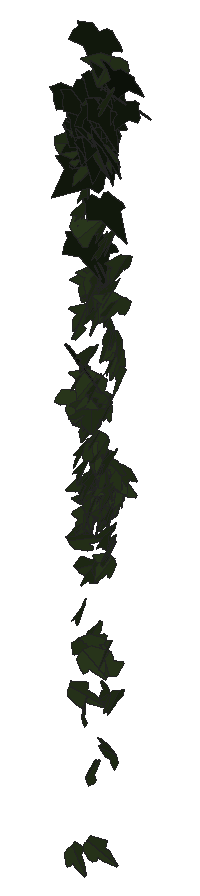
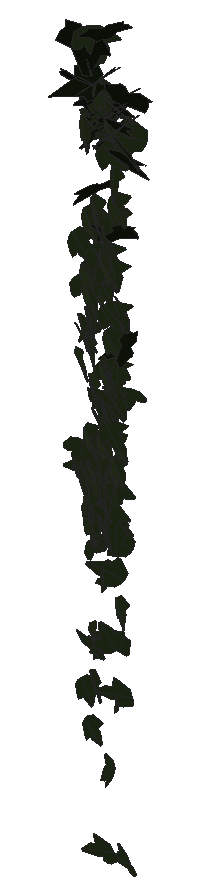
# SketchUp Ruby script. Lengths in inches.
U = 1.inch
M = Sketchup.active_model
def pt(a) = Geom::Point3d.new(a.map { |v| v * U })
def face(e, loops, mat)
  f = e.add_face(loops[0].map { |a| pt(a) })
  loops[1..].each { |l| e.add_face(l.map { |a| pt(a) }).erase! }
  f.material = f.back_material = mat if mat
  f
end
# faces: each face lists its corners as indices into pts; further lists are holes
def faces(e, pts, list, mat = nil) = list.each { |f| face(e, (f[0].is_a?(Array) ? f : [f]).map { |l| l.map { |i| pts[i] } }, mat) }
# xy, xz, yz: faces in a plane at the given z, y or x. An outline is a flat list of corners, or four numbers for a rectangle; further outlines are holes
def ring(l) = l.size == 4 ? [[l[0], l[1]], [l[2], l[1]], [l[2], l[3]], [l[0], l[3]]] : l.each_slice(2).to_a
def flat(e, list, mat, &to3) = list.each { |f| face(e, (f[0].is_a?(Array) ? f : [f]).map { |l| ring(l).map { |u, v| to3.(u, v) } }, mat) }
def xy(e, z, list, mat = nil) = flat(e, list, mat) { |x, y| [x, y, z] }
def xz(e, y, list, mat = nil) = flat(e, list, mat) { |x, z| [x, y, z] }
def yz(e, x, list, mat = nil) = flat(e, list, mat) { |y, z| [x, y, z] }
def lines(e, pts, list) = list.each { |a, b| e.add_line(pt(pts[a]), pt(pts[b])) }
# prism: a flat outline (further loops are holes) pulled along v
def prism(e, loops, v, mat = nil)
  f = face(e, loops, mat); d = Geom::Vector3d.new(v.map { |x| x * U })
  f.pushpull(f.normal.samedirection?(d) ? d.length : -d.length)
end
def box(e, o, s, mat = nil) = prism(e, [[o, [o[0] + s[0], o[1], o[2]], [o[0] + s[0], o[1] + s[1], o[2]], [o[0], o[1] + s[1], o[2]]]], [0, 0, s[2]], mat)
def at(x, y, z, deg = 0) = Geom::Transformation.translation(pt([x, y, z])) * Geom::Transformation.rotation(ORIGIN, Z_AXIS, deg.degrees)
def axes(o, x, y, z) = Geom::Transformation.new([*x, 0, *y, 0, *z, 0, *pt(o).to_a, 1])
def part(name) = M.definitions.add(name)
# library, detail: a bought-in or finely detailed component or shape, given as its bounding box
def library(name, o, s) = part(name).tap { |d| box(d.entities, o, s) }
def detail(e, o, s) = box(e.add_group.entities, o, s)
def put(e, d, t, mat = nil) = e.add_instance(d, t).tap { |i| i.material = mat if mat }
def group(e, t, mat = nil) = e.add_group.tap { |g| g.transformation = t; g.material = mat if mat }.entities
root = M.entities
M.materials.add("1026 AP 7946 SUNNY SIDE UP").color = [254, 231, 186]
M.materials.add("efeu1").color = [18, 25, 13]
M.materials.add("efeu2").color = [43, 57, 29]
c1 = part("ivyleaf_10")
p = [[0,0.5,-0.03],[-0.0625,2.02,-0.43],[-0.19,2.01,-0.46],[-0.54,1.05,-0.29],[-0.52,0.625,-0.18],[-0.83,0.76,-0.28],
  [-1.16,0.64,-0.33],[-1.15,0.33,-0.24],[-0.77,-0.39,0.02],[-0.3,-0.51,0.16],[0.04,-0.48,0.23],[-0.02,2.01,-0.4375],
  [-0.06,2.01,-0.43],[0.04,-0.49,0.23],[0.67,-0.49,0.14],[1.38,0.36,-0.2],[1.375,0.51,-0.24],[0.81,0.65,-0.19],
  [0.62,0.59,-0.15],[0.6,1.09,-0.28],[0.5,1.23,-0.31]]
faces(c1.entities,p,[[0,1,2,3,4,5,6,7,8,9,10],[11,12,0,13,14,15,16,17,18,19,20]],"efeu2")
c2 = part("ivyleaf_9")
p = [[1.54,2.16,1.25],[1.36,2.04,1.19],[-0.21,0.99,0.68],[-0.71,1.11,0.82],[-0.85,0.86,0.67],[-0.8,0.17,0.21],
  [-0.9,-0.01,0.1],[-0.67,-0.16,-0.02],[-0.08,-0.08,-0.05],[-0.03,-0.6,-0.4],[0.65,-0.88,-0.66],[0.83,-0.6,-0.49],
  [1.29,-0.42,-0.43],[1.8125,-0.07,-0.26],[1.21,0.44,0.15]]
faces(c2.entities,p,[[0,1,2,3,4,5,6,7,8,9,10,11,12,13,14]],"efeu1")
put(root,c1,axes([102.23,212.57,265.25],[0.00856,-0.04702,0.25643],[0.22762,0.20521,0.03784],[-0.32737,0.14145,0.03301]),"1026 AP 7946 SUNNY SIDE UP")
put(root,c2,axes([102.23,212.81,266.26],[-0.06893,-0.1302,-0.2167],[0.23021,0.15765,-0.1315],[0.31233,-0.14493,0.0491]),"1026 AP 7946 SUNNY SIDE UP")
put(root,c1,axes([102.46,212.81,257.53],[-0.08441,-0.19951,-0.06343],[0.03617,0.05635,-0.21239],[0.32579,-0.05795,0.00715]),"1026 AP 7946 SUNNY SIDE UP")
put(root,c1,axes([102.55,212.9,261.86],[-0.12366,-0.17588,0.12532],[-0.06753,-0.11507,-0.19904],[0.33033,-0.08937,0.00623]),"1026 AP 7946 SUNNY SIDE UP")
put(root,c1,axes([102.5,212.98,259.57],[-0.08704,-0.19196,0.06941],[-0.00761,-0.06969,-0.20573],[0.32037,-0.05381,0.01397]),"1026 AP 7946 SUNNY SIDE UP")
put(root,c1,axes([102.49,212.8,258.8],[0.03913,-0.20759,0.02258],[0.00037,-0.02323,-0.21551],[0.32842,0.02476,-0.00244]),"1026 AP 7946 SUNNY SIDE UP")
put(root,c1,axes([102.49,212.82,263.99],[0.01839,-0.23161,0.06678],[0.0176,-0.06562,-0.23917],[0.37833,0.01431,0.00788]),"1026 AP 7946 SUNNY SIDE UP")
put(root,c1,axes([102.46,212.875,258.34],[-0.19676,-0.16588,-0.03402],[0.07297,0.00464,-0.21117],[0.25545,-0.1291,0.03411]),"1026 AP 7946 SUNNY SIDE UP")
put(root,c2,axes([102.71,212.6,265.22],[-0.13705,0.20358,0.15107],[-0.11237,0.12739,-0.227],[-0.37706,-0.11196,0.01274]),"1026 AP 7946 SUNNY SIDE UP")
put(root,c1,axes([102.5,212.72,260.62],[-0.01401,-0.19739,-0.09822],[0.02439,0.09349,-0.20274],[0.34306,-0.01471,0.0104]),"1026 AP 7946 SUNNY SIDE UP")
put(root,c1,axes([102.52,212.96,257.97],[-0.31078,-0.0451,0.00766],[-0.00576,-0.0184,-0.20821],[0.07171,-0.19694,0.01648]),"1026 AP 7946 SUNNY SIDE UP")
put(root,c1,axes([102.42,212.61,260.19],[0.3303,0.05759,0.01292],[0.02587,-0.01397,-0.22372],[-0.08887,0.20995,-0.0171]),"1026 AP 7946 SUNNY SIDE UP")
put(root,c2,axes([102.4,212.9,265.5],[-0.04448,-0.22805,0.09015],[-0.00829,-0.0888,-0.2372],[0.38473,-0.02828,0.00531]),"1026 AP 7946 SUNNY SIDE UP")
put(root,c1,axes([102.52,212.67,255.95],[0.05359,-0.20151,-0.03586],[-0.00509,0.0336,-0.21033],[0.3212,0.03415,0.00265]),"1026 AP 7946 SUNNY SIDE UP")
put(root,c1,axes([102.5,212.91,258.3],[-0.22031,0.14566,-0.00796],[-0.01207,-0.0192,-0.20742],[-0.22911,-0.13905,0.01858]),"1026 AP 7946 SUNNY SIDE UP")
put(root,c1,axes([102.52,212.73,259.2],[0.07686,-0.20665,0.05315],[0.0099,-0.05271,-0.21899],[0.33522,0.04894,-0.00572]),"1026 AP 7946 SUNNY SIDE UP")
put(root,c1,axes([102.34,212.75,257.2],[-0.02932,-0.09159,0.1854],[0.1774,0.14577,0.08907],[-0.26421,0.10804,0.03923]),"1026 AP 7946 SUNNY SIDE UP")
put(root,c1,axes([102.29,212.71,250.92],[0.1527,-0.01544,0.19573],[0.27159,-0.08331,-0.09837],[0.12713,0.19652,-0.02496]),"1026 AP 7946 SUNNY SIDE UP")
put(root,c2,axes([102.36,212.76,265.53],[0.13548,-0.21942,-0.07672],[-0.01412,0.07491,-0.24169],[0.36345,0.0847,0.01921]),"1026 AP 7946 SUNNY SIDE UP")
put(root,c2,axes([102.68,212.7,264.87],[-0.40648,-0.0496,-0.00744],[0.01874,-0.02547,-0.26986],[0.07649,-0.25734,0.02656]),"1026 AP 7946 SUNNY SIDE UP")
put(root,c1,axes([102.58,212.78,260.07],[-0.07076,-0.19973,0.08069],[-0.01662,-0.07903,-0.21127],[0.33758,-0.04575,0.00651]),"1026 AP 7946 SUNNY SIDE UP")
put(root,c1,axes([102.52,212.52,261.57],[0.20033,-0.16147,0.11615],[-0.06386,0.11095,0.20992],[-0.30386,-0.12978,0.03246]),"1026 AP 7946 SUNNY SIDE UP")
put(root,c1,axes([102.57,212.94,257.67],[0.06609,-0.1916,-0.05329],[0.00491,0.0524,-0.20127],[0.31158,0.03982,0.01447]),"1026 AP 7946 SUNNY SIDE UP")
put(root,c2,axes([102.37,212.81,266.11],[0.06229,-0.24858,-0.02284],[0.05173,0.02605,-0.25642],[0.3888,0.03636,0.03778]),"1026 AP 7946 SUNNY SIDE UP")
put(root,c1,axes([102.57,212.71,257.79],[0.25266,-0.13027,-0.01838],[-0.03265,0.00149,-0.21274],[0.20399,0.16159,-0.01129]),"1026 AP 7946 SUNNY SIDE UP")
put(root,c2,axes([102.35,212.62,261.07],[0.26559,-0.17264,0.02342],[0.00585,-0.02945,-0.24831],[0.27395,0.168,-0.01741]),"1026 AP 7946 SUNNY SIDE UP")
put(root,c1,axes([102.57,212.92,265.62],[0.10291,-0.23379,0.03636],[0.02688,-0.03323,-0.25019],[0.37113,0.06724,0.00804]),"1026 AP 7946 SUNNY SIDE UP")
put(root,c2,axes([102.72,212.92,265.58],[-0.37095,-0.06087,0.02471],[-0.02725,-0.02972,-0.24992],[0.09941,-0.23529,0.02369]),"1026 AP 7946 SUNNY SIDE UP")
put(root,c1,axes([102.43,212.88,256.63],[-0.06672,-0.12304,0.17498],[0.14469,0.14558,0.13264],[-0.29734,0.09845,0.02528]),"1026 AP 7946 SUNNY SIDE UP")
put(root,c1,axes([102.58,212.875,258.43],[0.00164,-0.14497,0.14716],[0.03813,-0.14256,-0.14922],[0.31865,0.0178,0.0171]),"1026 AP 7946 SUNNY SIDE UP")
put(root,c1,axes([102.59,212.72,264.49],[0.06335,-0.22791,-0.05941],[0.04265,0.06133,-0.23511],[0.36669,0.03224,0.03761]),"1026 AP 7946 SUNNY SIDE UP")
put(root,c1,axes([102.55,212.84,255.21],[-0.08676,-0.19788,0.04812],[0.0137,0.04722,0.21186],[-0.31981,0.0557,-0.00398]),"1026 AP 7946 SUNNY SIDE UP")
put(root,c1,axes([102.58,212.69,258],[-0.10883,0.19768,-0.01227],[-0.00444,-0.01478,-0.21571],[-0.31147,-0.06886,0.00736]),"1026 AP 7946 SUNNY SIDE UP")
put(root,c1,axes([102.37,212.7,254.2],[0.06543,0.00414,0.20485],[0.3001,0.05624,-0.04202],[-0.08785,0.19519,0.009]),"1026 AP 7946 SUNNY SIDE UP")
put(root,c1,axes([102.63,212.93,262.76],[0.10702,-0.21342,0.05665],[0.00681,-0.05751,-0.23072],[0.34696,0.06696,-0.01295]),"1026 AP 7946 SUNNY SIDE UP")
put(root,c1,axes([102.76,212.43,253.97],[0.01141,0.00481,0.23076],[-0.22532,0.17235,0.00198],[-0.27077,-0.14322,0.00808]),"1026 AP 7946 SUNNY SIDE UP")
put(root,c1,axes([102.67,213,266.24],[-0.00842,-0.24534,0.02434],[-0.00042,-0.02502,-0.25295],[0.38777,-0.00536,0.00026]),"1026 AP 7946 SUNNY SIDE UP")
put(root,c1,axes([102.6875,212.7,252.61],[0.04701,-0.03625,0.21359],[-0.1336,0.18973,0.04786],[-0.30313,-0.08925,0.01203]),"1026 AP 7946 SUNNY SIDE UP")
put(root,c1,axes([102.68,212.79,262.62],[-0.14646,-0.2008,0.08033],[0.00287,-0.0869,-0.22551],[0.33935,-0.08593,0.03658]),"1026 AP 7946 SUNNY SIDE UP")
put(root,c1,axes([102.62,212.72,258.6],[0.11145,-0.16447,0.11129],[0.04665,-0.10558,-0.18468],[0.3067,0.07583,-0.01235]),"1026 AP 7946 SUNNY SIDE UP")
put(root,c1,axes([102.65,212.87,258.1],[0.09616,-0.19559,-0.02711],[0.01746,0.02976,-0.21],[0.30959,0.05907,0.02026]),"1026 AP 7946 SUNNY SIDE UP")
put(root,c1,axes([102.72,212.73,264.92],[-0.12234,-0.17888,0.15465],[-0.03452,-0.15298,-0.19908],[0.3666,-0.0741,0.03286]),"1026 AP 7946 SUNNY SIDE UP")
put(root,c1,axes([102.65,212.78,256.6875],[-0.02558,-0.1713,-0.12071],[0.04305,0.11376,-0.17604],[0.32262,-0.02876,0.01392]),"1026 AP 7946 SUNNY SIDE UP")
put(root,c1,axes([102.73,212.73,260.63],[-0.2183,-0.12036,0.12516],[-0.03949,-0.14122,-0.17355],[0.26676,-0.1194,0.07673]),"1026 AP 7946 SUNNY SIDE UP")
put(root,c1,axes([102.67,212.79,258.68],[-0.07659,-0.1915,-0.09256],[0.04523,0.08422,-0.20296],[0.3288,-0.05619,0.00636]),"1026 AP 7946 SUNNY SIDE UP")
put(root,c1,axes([102.7,212.91,258.48],[-0.13216,0.17537,0.06905],[-0.0787,0.04873,-0.19867],[-0.28395,-0.09513,0.02293]),"1026 AP 7946 SUNNY SIDE UP")
put(root,c1,axes([102.71,212.8,259.98],[-0.06404,-0.20034,0.08747],[0.0006,-0.0876,-0.21045],[0.34285,-0.03727,0.01671]),"1026 AP 7946 SUNNY SIDE UP")
put(root,c1,axes([102.68,212.98,258.92],[0.03709,-0.19635,-0.06696],[0.01879,0.06549,-0.20244],[0.32413,0.01867,0.0194]),"1026 AP 7946 SUNNY SIDE UP")
put(root,c1,axes([102.56,212.64,263.54],[0.14189,0.08335,-0.23864],[0.17076,0.20849,0.12184],[0.34818,-0.13622,0.0375]),"1026 AP 7946 SUNNY SIDE UP")
put(root,c1,axes([102.71,212.7,261.2],[0.00422,-0.21412,0.05875],[-0.00307,-0.05827,-0.22092],[0.3489,0.00208,-0.00266]),"1026 AP 7946 SUNNY SIDE UP")
put(root,c1,axes([102.87,212.75,265.86],[-0.26308,-0.01154,0.1826],[-0.19966,-0.16261,-0.13528],[0.19545,-0.18164,0.10759]),"1026 AP 7946 SUNNY SIDE UP")
put(root,c1,axes([102.68,212.78,260.56],[0.18109,-0.18219,0.03066],[0.00784,-0.03321,-0.22181],[0.29044,0.11449,-0.01312]),"1026 AP 7946 SUNNY SIDE UP")
put(root,c1,axes([102.62,212.79,257.98],[0.03838,-0.13807,0.15475],[0.10594,-0.13816,-0.14218],[0.30379,0.06563,0.03003]),"1026 AP 7946 SUNNY SIDE UP")
put(root,c1,axes([102.73,212.93,258.2],[-0.15247,-0.17258,0.05742],[0.00322,-0.06533,-0.20155],[0.28563,-0.09139,0.03293]),"1026 AP 7946 SUNNY SIDE UP")
put(root,c1,axes([102.66,212.96,257.99],[0.19469,-0.15049,0.06094],[0.04437,-0.05434,-0.20069],[0.25085,0.12641,-0.0118]),"1026 AP 7946 SUNNY SIDE UP")
put(root,c2,axes([102.5,212.8,265.74],[0.15521,-0.22651,-0.04144],[0.02425,0.04881,-0.25194],[0.36057,0.09422,0.03478]),"1026 AP 7946 SUNNY SIDE UP")
put(root,c1,axes([102.73,212.92,258.76],[0.10799,-0.19417,-0.04235],[-0.01765,0.03846,-0.21194],[0.31122,0.06956,0.00267]),"1026 AP 7946 SUNNY SIDE UP")
put(root,c2,axes([102.53,212.73,265.8125],[0.11394,-0.22686,-0.07785],[0.01368,0.08008,-0.24276],[0.3751,0.06599,0.0325]),"1026 AP 7946 SUNNY SIDE UP")
put(root,c1,axes([102.58,212.6875,255.26],[-0.19898,-0.0896,-0.15316],[0.21618,0.05956,-0.15773],[0.16551,-0.18552,0.02188]),"1026 AP 7946 SUNNY SIDE UP")
put(root,c1,axes([102.79,212.92,260.11],[0.27629,-0.09475,-0.10495],[-0.12058,0.06994,-0.20395],[0.18179,0.1904,0.02423]),"1026 AP 7946 SUNNY SIDE UP")
put(root,c1,axes([102.76,212.91,258.23],[-0.09171,-0.19668,0.03391],[-0.00924,-0.03374,-0.2115],[0.31371,-0.05849,0.00368]),"1026 AP 7946 SUNNY SIDE UP")
put(root,c1,axes([102.71,212.74,258.6],[0.0876,-0.18637,0.10523],[0.03619,-0.10078,-0.20089],[0.33302,0.05998,-0.00585]),"1026 AP 7946 SUNNY SIDE UP")
put(root,c1,axes([102.66,212.77,262.56],[-0.08524,0.2035,-0.09458],[0.03031,-0.09105,-0.21744],[-0.35049,-0.05737,0.0042]),"1026 AP 7946 SUNNY SIDE UP")
put(root,c1,axes([102.75,212.66,259.96],[-0.20954,-0.17551,-0.01307],[0.022,0.00404,-0.22682],[0.2757,-0.13371,0.00817]),"1026 AP 7946 SUNNY SIDE UP")
put(root,c2,axes([102.65,212.97,267.46],[-0.12631,-0.23978,-0.03145],[0.02137,0.02621,-0.26032],[0.37921,-0.08134,0.00419]),"1026 AP 7946 SUNNY SIDE UP")
put(root,c1,axes([102.74,212.92,257.73],[0.12867,-0.18449,-0.03139],[-0.00023,0.03206,-0.20731],[0.29376,0.08083,0.01359]),"1026 AP 7946 SUNNY SIDE UP")
put(root,c1,axes([102.74,212.77,259.43],[0.13115,-0.19724,0.06609],[0.02224,-0.06479,-0.22067],[0.32593,0.08379,-0.01154]),"1026 AP 7946 SUNNY SIDE UP")
put(root,c2,axes([102.9,212.84,266.0625],[-0.37854,0.06006,-0.04672],[0.05544,-0.04554,-0.25331],[-0.10491,-0.24077,0.03471]),"1026 AP 7946 SUNNY SIDE UP")
put(root,c1,axes([102.75,212.6875,262.93],[-0.22577,0.17996,0.00734],[-0.02609,-0.00544,-0.23661],[-0.28193,-0.14361,0.01601]),"1026 AP 7946 SUNNY SIDE UP")
put(root,c1,axes([102.79,212.84,262.37],[-0.03703,-0.22143,0.0561],[-0.00398,-0.05575,-0.22971],[0.35901,-0.02345,0.00324]),"1026 AP 7946 SUNNY SIDE UP")
put(root,c1,axes([102.8,212.93,258.42],[0.02664,-0.20754,0.00046],[-0.00394,-0.00183,-0.21452],[0.32633,0.01692,-0.00263]),"1026 AP 7946 SUNNY SIDE UP")
put(root,c1,axes([102.84,212.875,258.2],[-0.20963,-0.12167,0.09641],[-0.03953,-0.10583,-0.17796],[0.23878,-0.12434,0.05518]),"1026 AP 7946 SUNNY SIDE UP")
put(root,c1,axes([102.8,212.74,260.57],[0.07591,-0.22124,0.01977],[0.00117,-0.02076,-0.23338],[0.34936,0.04814,-0.00352]),"1026 AP 7946 SUNNY SIDE UP")
put(root,c1,axes([102.73,212.79,265.73],[0.02735,0.24073,-0.03026],[-0.00049,-0.03079,-0.24882],[-0.3816,0.0173,-0.00185]),"1026 AP 7946 SUNNY SIDE UP")
put(root,c2,axes([102.61,213.01,266.52],[0.13111,-0.22167,-0.07749],[-0.00239,0.07801,-0.24218],[0.36744,0.07961,0.02608]),"1026 AP 7946 SUNNY SIDE UP")
put(root,c2,axes([102.66,212.72,263.4],[-0.13163,-0.19265,-0.13659],[0.11378,0.11136,-0.21488],[0.34865,-0.10907,0.01856]),"1026 AP 7946 SUNNY SIDE UP")
put(root,c1,axes([102.79,212.85,261.9375],[0.17923,-0.19006,0.03809],[0.01234,-0.03958,-0.22812],[0.30453,0.11346,-0.01317]),"1026 AP 7946 SUNNY SIDE UP")
put(root,c1,axes([102.81,212.71,262.98],[-0.25331,0.16471,0.00751],[-0.02265,-0.00522,-0.23694],[-0.25819,-0.16114,0.01342]),"1026 AP 7946 SUNNY SIDE UP")
put(root,c2,axes([102.69,212.76,265.2],[-0.00528,-0.20134,0.14343],[0.01058,-0.14041,-0.20813],[0.38579,0.0011,0.00767]),"1026 AP 7946 SUNNY SIDE UP")
put(root,c1,axes([102.875,212.69,262.84],[-0.15151,-0.18668,0.09676],[0.0096,-0.10701,-0.21091],[0.3292,-0.08279,0.05068]),"1026 AP 7946 SUNNY SIDE UP")
put(root,c2,axes([102.84,212.77,265.86],[-0.31522,-0.10676,-0.09244],[0.13339,0.03002,-0.23345],[0.17328,-0.21732,0.01156]),"1026 AP 7946 SUNNY SIDE UP")
put(root,c1,axes([102.85,212.75,259.11],[0.0831,-0.19818,0.07971],[0.02198,-0.07748,-0.21166],[0.33446,0.05433,-0.00589]),"1026 AP 7946 SUNNY SIDE UP")
put(root,c1,axes([102.92,212.8,262.84],[-0.08243,-0.19292,0.11979],[-0.02057,-0.1177,-0.206],[0.35449,-0.05169,0.0159]),"1026 AP 7946 SUNNY SIDE UP")
put(root,c1,axes([102.84,212.875,262.74],[-0.1288,0.21402,-0.01123],[-0.00914,-0.01518,-0.23591],[-0.33694,-0.0814,0.01069]),"1026 AP 7946 SUNNY SIDE UP")
put(root,c1,axes([102.62,212.85,251.09],[0.12536,0.0171,0.1931],[0.29161,0.027,-0.08369],[-0.04964,0.20181,-0.00395]),"1026 AP 7946 SUNNY SIDE UP")
put(root,c1,axes([102.9,212.86,263.82],[0.09975,-0.23282,0.01093],[-0.00365,-0.013,-0.2486],[0.36654,0.06323,-0.00545]),"1026 AP 7946 SUNNY SIDE UP")
put(root,c1,axes([102.82,212.6,259.3],[0.07151,0.20868,-0.02843],[-0.00287,-0.02905,-0.22015],[-0.33122,0.04531,-0.00423]),"1026 AP 7946 SUNNY SIDE UP")
put(root,c1,axes([102.92,212.95,257.92],[-0.08065,-0.18547,0.06598],[-0.00828,-0.06596,-0.19825],[0.30897,-0.05018,0.01191]),"1026 AP 7946 SUNNY SIDE UP")
put(root,c1,axes([102.84,212.71,262.7],[0.09979,-0.16798,0.15633],[0.07993,-0.14402,-0.18581],[0.34789,0.08127,-0.00215]),"1026 AP 7946 SUNNY SIDE UP")
put(root,c1,axes([102.89,212.84,258.14],[-0.01939,0.16865,0.11743],[-0.05056,0.11019,-0.17234],[-0.3152,-0.02805,0.02042]),"1026 AP 7946 SUNNY SIDE UP")
put(root,c1,axes([102.78,212.54,255.11],[0.10724,0.18247,0.11419],[0.07215,0.10001,-0.19997],[-0.327,0.0819,-0.00667]),"1026 AP 7946 SUNNY SIDE UP")
put(root,c1,axes([102.86,212.92,260.16],[0.2365,-0.15293,0.06654],[0.05514,-0.05712,-0.22081],[0.25569,0.15377,-0.01393]),"1026 AP 7946 SUNNY SIDE UP")
put(root,c1,axes([102.95,212.92,257.57],[-0.01243,-0.20224,0.01365],[-0.00091,-0.01439,-0.20859],[0.31881,-0.00792,-0.00006]),"1026 AP 7946 SUNNY SIDE UP")
put(root,c1,axes([102.91,212.88,259.05],[0.11807,-0.16145,0.10452],[0.0655,-0.09352,-0.18397],[0.29337,0.08586,-0.00099]),"1026 AP 7946 SUNNY SIDE UP")
put(root,c1,axes([103.04,212.72,254.35],[0.11757,-0.12507,-0.15243],[-0.09485,0.13489,-0.14879],[0.2886,0.09528,0.0132]),"1026 AP 7946 SUNNY SIDE UP")
put(root,c2,axes([102.86,212.8,265.96],[-0.08878,-0.2345,-0.06974],[0.03045,0.06359,-0.24808],[0.38199,-0.05957,0.00356]),"1026 AP 7946 SUNNY SIDE UP")
put(root,c1,axes([102.97,212.89,258.64],[0.11987,-0.18538,0.04798],[0.01243,-0.04817,-0.20648],[0.3007,0.07589,-0.01059]),"1026 AP 7946 SUNNY SIDE UP")
put(root,c1,axes([103.07,212.78,267.12],[-0.29454,-0.15669,0.08444],[-0.05256,-0.08715,-0.24817],[0.2737,-0.18536,0.0432]),"1026 AP 7946 SUNNY SIDE UP")
put(root,c1,axes([103,212.92,257.97],[0.01741,-0.2019,-0.0233],[0.0014,0.02155,-0.20817],[0.31926,0.01092,0.00218]),"1026 AP 7946 SUNNY SIDE UP")
put(root,c1,axes([103.02,212.65,263.51],[0.06762,-0.23409,-0.05946],[-0.01792,0.05524,-0.24487],[0.37819,0.04447,-0.00097]),"1026 AP 7946 SUNNY SIDE UP")
put(root,c1,axes([102.93,212.59,265.42],[-0.36709,0.07603,-0.07197],[0.09232,-0.04562,-0.25197],[-0.13412,-0.2395,0.02355]),"1026 AP 7946 SUNNY SIDE UP")
put(root,c1,axes([103,212.67,259.48],[0.22215,-0.16082,-0.00399],[-0.01796,-0.00611,-0.22018],[0.25227,0.14118,-0.01217]),"1026 AP 7946 SUNNY SIDE UP")
put(root,c1,axes([103,212.86,258.07],[0.09288,-0.19118,-0.03764],[0.00446,0.03789,-0.20543],[0.3057,0.05753,0.01443]),"1026 AP 7946 SUNNY SIDE UP")
put(root,c1,axes([103.03,212.93,262.53],[0.02402,-0.22226,0.05671],[-0.00464,-0.05662,-0.22974],[0.36049,0.01408,-0.00674]),"1026 AP 7946 SUNNY SIDE UP")
put(root,c2,axes([102.86,212.73,265.73],[0.0322,-0.226,0.08995],[0.00733,-0.08853,-0.23427],[0.38162,0.02077,-0.00309]),"1026 AP 7946 SUNNY SIDE UP")
put(root,c1,axes([103.03,212.9,263.59],[0.03156,-0.23815,0.01445],[0.00107,-0.01538,-0.2463],[0.37524,0.02008,-0.00052]),"1026 AP 7946 SUNNY SIDE UP")
put(root,c1,axes([102.99,212.92,261.43],[0.04944,0.1416,-0.17655],[-0.04809,-0.1695,-0.15035],[-0.34722,0.04364,-0.00432]),"1026 AP 7946 SUNNY SIDE UP")
put(root,c1,axes([103.04,212.83,261.68],[0.16936,-0.18409,-0.09592],[-0.02795,0.0952,-0.21697],[0.32243,0.10494,0.03157]),"1026 AP 7946 SUNNY SIDE UP")
put(root,c2,axes([102.86,212.91,265.26],[0.05967,-0.21608,0.10745],[0.00809,-0.10608,-0.2263],[0.37804,0.03638,-0.01212]),"1026 AP 7946 SUNNY SIDE UP")
put(root,c1,axes([103.04,212.9,262.15],[0.04871,-0.2292,0.01393],[-0.00507,-0.01539,-0.2383],[0.36111,0.0307,-0.00522]),"1026 AP 7946 SUNNY SIDE UP")
put(root,c2,axes([102.86,212.81,264.21],[0.06171,-0.21448,-0.11301],[0.01731,0.1114,-0.22216],[0.37753,0.02995,0.02866]),"1026 AP 7946 SUNNY SIDE UP")
put(root,c1,axes([102.98,212.8125,255.27],[0.14988,-0.14846,0.10905],[0.06355,-0.10024,-0.18147],[0.28036,0.10209,-0.01716]),"1026 AP 7946 SUNNY SIDE UP")
put(root,c1,axes([103.06,212.85,261.09],[0.09414,-0.20703,-0.06325],[-0.024,0.05827,-0.22168],[0.33818,0.06177,0.00187]),"1026 AP 7946 SUNNY SIDE UP")
put(root,c2,axes([102.8,213.01,266.375],[0.3627,-0.08964,-0.00331],[0.03208,0.05972,-0.24618],[0.13732,0.22282,0.06626]),"1026 AP 7946 SUNNY SIDE UP")
put(root,c1,axes([103.07,212.73,260.21],[0.08705,-0.19836,-0.07306],[-0.02382,0.06822,-0.21173],[0.32978,0.05729,0.00399]),"1026 AP 7946 SUNNY SIDE UP")
put(root,c1,axes([103.11,212.6875,254.9],[0.26967,-0.03636,0.11484],[-0.16363,0.0446,0.17985],[-0.08563,-0.19974,0.01799]),"1026 AP 7946 SUNNY SIDE UP")
put(root,c1,axes([103.03,212.78,256.99],[-0.084,-0.10036,0.17797],[0.05842,-0.18123,-0.09737],[0.30945,0.00697,0.06669]),"1026 AP 7946 SUNNY SIDE UP")
put(root,c1,axes([103.13,212.9,262.26],[-0.18446,-0.15124,0.13356],[-0.04564,-0.13683,-0.19104],[0.31078,-0.10986,0.05122]),"1026 AP 7946 SUNNY SIDE UP")
put(root,c1,axes([103.07,212.71,257.59],[0.01811,-0.19561,-0.06437],[0.01479,0.06191,-0.2011],[0.32202,0.00816,0.01286]),"1026 AP 7946 SUNNY SIDE UP")
put(root,c1,axes([103,212.9,258.93],[-0.25934,0.10171,-0.07322],[0.07627,-0.057,-0.19871],[-0.18015,-0.17055,0.02128]),"1026 AP 7946 SUNNY SIDE UP")
put(root,c1,axes([103.09,212.93,254.28],[-0.04175,-0.19612,0.04536],[-0.0023,-0.04535,-0.20409],[0.31643,-0.02621,0.0045]),"1026 AP 7946 SUNNY SIDE UP")
put(root,c1,axes([103.09,212.93,265.4],[0.06122,-0.23834,-0.03599],[0.02096,0.0361,-0.24782],[0.37788,0.03661,0.01958]),"1026 AP 7946 SUNNY SIDE UP")
put(root,c1,axes([103.14,212.81,258.7],[0.1745,0.1073,-0.13766],[-0.15168,-0.09334,-0.15957],[-0.22362,0.14704,0.00082]),"1026 AP 7946 SUNNY SIDE UP")
put(root,c1,axes([103.07,212.76,258.77],[0.09632,0.19537,0.0168],[-0.0526,0.02612,-0.20679],[-0.3036,0.05746,0.04116]),"1026 AP 7946 SUNNY SIDE UP")
put(root,c1,axes([103.12,212.75,258.83],[0.29046,-0.0935,-0.05499],[-0.08258,0.01308,-0.21287],[0.14731,0.19169,-0.01091]),"1026 AP 7946 SUNNY SIDE UP")
put(root,c1,axes([103.14,212.76,261.53],[0.11277,-0.19964,-0.09753],[-0.04043,0.09011,-0.21793],[0.34429,0.07597,0.00635]),"1026 AP 7946 SUNNY SIDE UP")
put(root,c1,axes([103.11,212.79,259.19],[0.06824,-0.20004,0.06021],[0.00709,-0.05994,-0.21107],[0.32813,0.0429,-0.00796]),"1026 AP 7946 SUNNY SIDE UP")
put(root,c1,axes([103.05,212.8125,258.75],[-0.00854,0.19821,-0.05939],[0.00534,-0.0587,-0.20461],[-0.32504,-0.00617,-0.0018]),"1026 AP 7946 SUNNY SIDE UP")
put(root,c2,axes([102.95,212.68,266.21],[0.09383,-0.24251,-0.03113],[-0.02321,0.02605,-0.257],[0.38331,0.06094,-0.00794]),"1026 AP 7946 SUNNY SIDE UP")
put(root,c1,axes([103.24,212.59,253.29],[0.13743,-0.01946,-0.18966],[-0.17704,0.15588,-0.07117],[0.23086,0.13113,0.05833]),"1026 AP 7946 SUNNY SIDE UP")
put(root,c1,axes([103.17,212.89,261.44],[0.17669,-0.15312,-0.12935],[-0.06852,0.1207,-0.19245],[0.30285,0.11664,0.03192]),"1026 AP 7946 SUNNY SIDE UP")
put(root,c1,axes([103.13,212.67,266.51],[0.10253,-0.24461,0.03079],[-0.00137,-0.03258,-0.26081],[0.38775,0.06456,-0.00906]),"1026 AP 7946 SUNNY SIDE UP")
put(root,c1,axes([103.15,212.74,257.39],[0.10373,-0.18834,-0.04285],[-0.01771,0.03899,-0.20535],[0.30241,0.06689,0.00267]),"1026 AP 7946 SUNNY SIDE UP")
put(root,c1,axes([103.15,212.55,257.23],[0.13407,-0.09727,0.19878],[-0.11899,0.18148,0.12939],[-0.31908,-0.10854,0.03528]),"1026 AP 7946 SUNNY SIDE UP")
put(root,c1,axes([103.14,212.77,258.54],[0.04146,-0.17929,0.12258],[0.03765,-0.11772,-0.1873],[0.33715,0.03519,0.00584]),"1026 AP 7946 SUNNY SIDE UP")
put(root,c2,axes([102.95,212.71,265.59],[0.12929,-0.22034,0.08637],[0.03636,-0.08215,-0.24267],[0.36961,0.08516,-0.00634]),"1026 AP 7946 SUNNY SIDE UP")
put(root,c1,axes([103.11,212.89,258.55],[0.32129,0.03805,-0.00091],[-0.00192,0.00055,-0.21411],[-0.05982,0.20433,0.00198]),"1026 AP 7946 SUNNY SIDE UP")
put(root,c1,axes([103.17,212.97,260.75],[0.16107,-0.1914,0.03025],[0.01552,-0.02925,-0.22375],[0.30434,0.10279,-0.0046]),"1026 AP 7946 SUNNY SIDE UP")
put(root,c2,axes([103.22,212.97,266.27],[-0.35443,-0.05895,-0.09012],[0.14923,-0.025,-0.23562],[0.0714,-0.24037,0.0451]),"1026 AP 7946 SUNNY SIDE UP")
put(root,c2,axes([103.22,212.71,267.01],[0.3242,0.04974,-0.17095],[-0.2406,-0.06959,-0.21738],[-0.12863,0.25554,-0.02426]),"1026 AP 7946 SUNNY SIDE UP")
put(root,c1,axes([103.15,212.94,258.34],[0.21395,-0.15211,0.0333],[0.04107,-0.02115,-0.2103],[0.24134,0.13845,0.00627]),"1026 AP 7946 SUNNY SIDE UP")
put(root,c1,axes([103.13,212.9,261.1875],[0.27653,-0.126,0.065],[0.061,-0.05489,-0.22213],[0.21353,0.17885,-0.02072]),"1026 AP 7946 SUNNY SIDE UP")
put(root,c1,axes([103.22,212.88,258.94],[-0.31235,0.0607,0.00764],[-0.01954,-0.01657,-0.21314],[-0.09408,-0.19808,0.0189]),"1026 AP 7946 SUNNY SIDE UP")
put(root,c1,axes([103.23,212.95,263.09],[-0.04971,-0.21016,0.09722],[0.00466,-0.09682,-0.2189],[0.36299,-0.02754,0.01612]),"1026 AP 7946 SUNNY SIDE UP")
